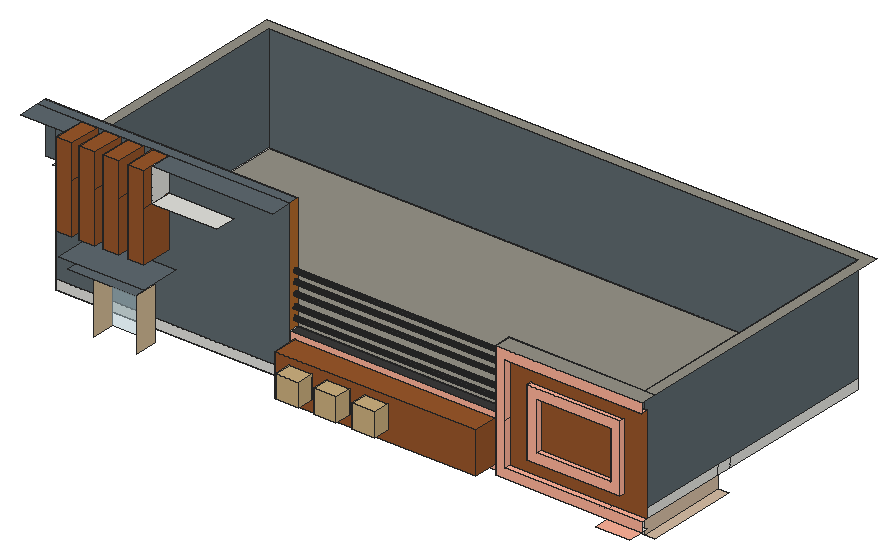
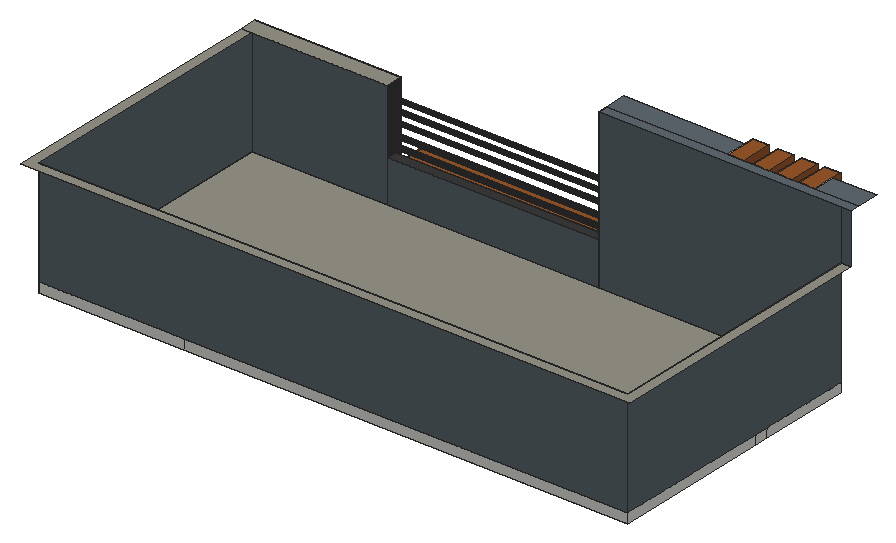
# SketchUp Ruby script. Lengths in inches.
U = 1.inch
M = Sketchup.active_model
def pt(a) = Geom::Point3d.new(a.map { |v| v * U })
def face(e, loops, mat)
  f = e.add_face(loops[0].map { |a| pt(a) })
  loops[1..].each { |l| e.add_face(l.map { |a| pt(a) }).erase! }
  f.material = f.back_material = mat if mat
  f
end
# faces: each face lists its corners as indices into pts; further lists are holes
def faces(e, pts, list, mat = nil) = list.each { |f| face(e, (f[0].is_a?(Array) ? f : [f]).map { |l| l.map { |i| pts[i] } }, mat) }
# xy, xz, yz: faces in a plane at the given z, y or x. An outline is a flat list of corners, or four numbers for a rectangle; further outlines are holes
def ring(l) = l.size == 4 ? [[l[0], l[1]], [l[2], l[1]], [l[2], l[3]], [l[0], l[3]]] : l.each_slice(2).to_a
def flat(e, list, mat, &to3) = list.each { |f| face(e, (f[0].is_a?(Array) ? f : [f]).map { |l| ring(l).map { |u, v| to3.(u, v) } }, mat) }
def xy(e, z, list, mat = nil) = flat(e, list, mat) { |x, y| [x, y, z] }
def xz(e, y, list, mat = nil) = flat(e, list, mat) { |x, z| [x, y, z] }
def yz(e, x, list, mat = nil) = flat(e, list, mat) { |y, z| [x, y, z] }
def lines(e, pts, list) = list.each { |a, b| e.add_line(pt(pts[a]), pt(pts[b])) }
# prism: a flat outline (further loops are holes) pulled along v
def prism(e, loops, v, mat = nil)
  f = face(e, loops, mat); d = Geom::Vector3d.new(v.map { |x| x * U })
  f.pushpull(f.normal.samedirection?(d) ? d.length : -d.length)
end
def box(e, o, s, mat = nil) = prism(e, [[o, [o[0] + s[0], o[1], o[2]], [o[0] + s[0], o[1] + s[1], o[2]], [o[0], o[1] + s[1], o[2]]]], [0, 0, s[2]], mat)
def at(x, y, z, deg = 0) = Geom::Transformation.translation(pt([x, y, z])) * Geom::Transformation.rotation(ORIGIN, Z_AXIS, deg.degrees)
def axes(o, x, y, z) = Geom::Transformation.new([*x, 0, *y, 0, *z, 0, *pt(o).to_a, 1])
def part(name) = M.definitions.add(name)
# library, detail: a bought-in or finely detailed component or shape, given as its bounding box
def library(name, o, s) = part(name).tap { |d| box(d.entities, o, s) }
def detail(e, o, s) = box(e.add_group.entities, o, s)
def put(e, d, t, mat = nil) = e.add_instance(d, t).tap { |i| i.material = mat if mat }
def group(e, t, mat = nil) = e.add_group.tap { |g| g.transformation = t; g.material = mat if mat }.entities
root = M.entities
M.materials.add("[Color B02]").color = [255, 178, 153]
M.materials.add("[Color C02]").color = [255, 204, 153]
M.materials.add("[Color M07]").color = [58, 58, 58]
M.materials.add("[Formica Beige]").color = [211, 187, 149]
M.materials.add("[Formica Graystone]").color = [149, 146, 135]
M.materials.add("[Formica Laminate Light]").color = [213, 189, 164]
M.materials.add("[Formica Speckled Grey]").color = [94, 105, 111]
M.materials.add("[Translucent Glass Safety]").color = [204, 235, 244]
M.materials["[Translucent Glass Safety]"].alpha = 0.5
M.materials.add("[Wood Bamboo]").color = [177, 105, 43]
M.materials.add("[Wood Cherry Original]").color = [152, 86, 42]
M.materials.add("[Wood Floor Light]").color = [204, 176, 127]
xy(root,228.95,[[257.7,166.38,329.95,178.72]])
xy(root,232,[[391.28,166.38,447.72,178.72]])
xy(root,237.86,[[524.83,85.74,533.83,166.38]],"[Formica Laminate Light]")
xy(root,249,[[504.33,70.93,533.83,76.74],[9,166.38,524.83,178.72],[9,178.72,524.83,319.17]])
xy(root,249,[[504.33,57.99,533.83,70.93],[9,85.74,524.83,166.38]],"[Color B02]")
xy(root,249,[[405.9,70.93,405.9,76.74,221.09,76.74,221.09,85.74,504.33,85.74,504.33,70.93]],"[Color C02]")
xy(root,253.72,[[225.3125,54.93,401.17,76.74]],"[Wood Cherry Original]")
xy(root,257.375,[[9,85.74,524.83,319.17]],"[Formica Graystone]")
xy(root,257.39,[[414.29,70.93,504.33,76.74],[504.33,70.93,533.83,76.74]],"[Color B02]")
xy(root,263.47,[[238.12,54.93,258.18,69.68],[271.06,54.93,291.12,69.68],[304.56,54.93,324.62,69.68],[238.12,69.68,258.18,76.74],[271.06,69.68,291.12,76.74],
  [304.56,69.68,324.62,76.74]])
xy(root,263.47,[[238.12,40.06,258.18,54.93],[271.06,40.06,291.12,54.93],[304.56,40.06,324.62,54.93]],"[Wood Floor Light]")
xy(root,269.68,[[432.09,72.56,513.84,76.74]],"[Color B02]")
xy(root,278.24,[[440.64,72.56,505.28,76.74]],"[Color B02]")
xy(root,283.54,[[238.12,54.93,258.18,69.68],[271.06,54.93,291.12,69.68],[304.56,54.93,324.62,69.68],[238.12,69.68,258.18,76.74],[271.06,69.68,291.12,76.74],
  [304.56,69.68,324.62,76.74]])
xy(root,283.54,[[238.12,40.06,258.18,54.93],[271.06,40.06,291.12,54.93],[304.56,40.06,324.62,54.93]],"[Wood Floor Light]")
xy(root,289.38,[[65.18,56.99,102.75,76.74]],"[Formica Beige]")
xy(root,289.78,[[225.3125,54.93,401.17,76.74]],"[Wood Cherry Original]")
xy(root,294.5,[[221.09,76.74,405.9,85.74]],"[Color M07]")
xy(root,300.29,[[54.27,41.68,113.66,56.99]],"[Formica Speckled Grey]")
xy(root,307.5625,[[47,41.68,120.93,76.74]],"[Formica Speckled Grey]")
xy(root,320.12,[[440.64,72.56,505.28,76.74]],"[Color B02]")
xy(root,321.4375,[[38.68,48.99,52.74,76.74],[58.74,48.99,72.8,76.74],[79.11,48.99,93.18,76.74],[100.98,48.99,115.05,76.74]],"[Wood Cherry Original]")
xy(root,328.68,[[432.09,72.56,513.84,76.74]],"[Color B02]")
xy(root,342.48,[[414.29,70.93,533.83,76.74]],"[Color B02]")
xy(root,350.875,[[405.9,70.93,533.83,85.74],[0,85.74,9,85.74,9,319.17,524.83,319.17,524.83,85.74,533.83,85.74,533.83,328.17,0,328.17]],"[Formica Graystone]")
xy(root,365.9375,[[28.26,57.99,38.68,76.74],[115.05,57.99,172.2,76.74]])
xy(root,395.1875,[[0,57.99,38.68,76.74],[115.05,57.99,221.09,76.74],[0,76.74,221.09,85.74]],"[Formica Speckled Grey]")
xy(root,395.1875,[[38.68,48.99,52.74,76.74],[58.74,48.99,72.8,76.74],[79.11,48.99,93.18,76.74],[100.98,48.99,115.05,76.74]],"[Wood Cherry Original]")
xz(root,40.06,[[238.12,263.47,258.18,283.54],[271.06,263.47,291.12,283.54],[304.56,263.47,324.62,283.54]],"[Wood Floor Light]")
xz(root,48.99,[[38.68,321.4375,52.74,395.1875],[58.74,321.4375,72.8,395.1875],[79.11,321.4375,93.18,395.1875],[100.98,321.4375,115.05,395.1875]],"[Wood Cherry Original]")
xz(root,54.93,[[[225.3125,253.72,401.17,289.78],[238.12,263.47,258.18,283.54],[271.06,263.47,291.12,283.54],[304.56,263.47,324.62,283.54]]],"[Wood Cherry Original]")
xz(root,69.68,[[238.12,263.47,258.18,283.54],[271.06,263.47,291.12,283.54],[304.56,263.47,324.62,283.54]])
xz(root,70.93,[[405.9,249,533.83,249,533.83,257.39,414.29,257.39,414.29,342.48,533.83,342.48,533.83,350.875,405.9,350.875]],"[Color B02]")
xz(root,72.56,[[[432.09,269.68,513.84,328.68],[440.64,278.24,505.28,320.12]]],"[Color B02]")
xz(root,76.74,[[238.12,263.47,258.18,283.54],[271.06,263.47,291.12,283.54],[304.56,263.47,324.62,283.54],[38.68,321.4375,52.74,395.1875],[58.74,321.4375,72.8,395.1875],
  [79.11,321.4375,93.18,395.1875],[100.98,321.4375,115.05,395.1875]])
xz(root,76.74,[[[221.09,249,405.9,294.5],[225.3125,253.72,401.17,289.78]]],"[Color B02]")
xz(root,76.74,[[52.74,365.9375,58.74,395.1875],[72.8,365.9375,79.11,395.1875],[93.18,365.9375,100.98,395.1875]],"[Formica Speckled Grey]")
xz(root,76.74,[[65.18,244.12,102.75,289.38]],"[Translucent Glass Safety]")
xz(root,76.74,[[[414.29,257.39,533.83,342.48],[432.09,269.68,513.84,328.68]],[440.64,278.24,505.28,320.12]],"[Wood Cherry Original]")
xz(root,85.74,[[504.33,237.86,524.83,249],[9,249,221.09,257.375],[221.09,249,524.83,257.375]])
xz(root,85.74,[[9,257.375,221.09,395.1875],[221.09,257.375,405.9,294.5],[405.9,257.375,524.83,350.875],[0,350.875,9,395.1875]],"[Formica Speckled Grey]")
xz(root,319.17,[[9,249,398.15,257.375],[398.15,249,524.83,257.375]])
xz(root,319.17,[[9,257.375,524.83,350.875]],"[Formica Speckled Grey]")
yz(root,9,[[85.74,249,166.38,257.375],[166.38,249,178.72,257.375],[178.72,249,319.17,257.375]])
yz(root,9,[[85.74,257.375,319.17,350.875]],"[Formica Speckled Grey]")
yz(root,38.68,[[57.99,365.9375,76.74,395.1875]])
yz(root,38.68,[[48.99,321.4375,76.74,365.9375],[48.99,365.9375,57.99,395.1875]],"[Wood Cherry Original]")
yz(root,52.74,[[48.99,321.4375,76.74,365.9375],[48.99,365.9375,76.74,395.1875]],"[Wood Cherry Original]")
yz(root,58.74,[[48.99,321.4375,76.74,365.9375],[48.99,365.9375,76.74,395.1875]],"[Wood Cherry Original]")
yz(root,65.18,[[56.99,244.12,76.74,289.38]],"[Formica Beige]")
yz(root,72.8,[[48.99,321.4375,76.74,365.9375],[48.99,365.9375,76.74,395.1875]],"[Wood Cherry Original]")
yz(root,79.11,[[48.99,321.4375,76.74,365.9375],[48.99,365.9375,76.74,395.1875]],"[Wood Cherry Original]")
yz(root,93.18,[[48.99,321.4375,76.74,365.9375],[48.99,365.9375,76.74,395.1875]],"[Wood Cherry Original]")
yz(root,100.98,[[48.99,321.4375,76.74,365.9375],[48.99,365.9375,76.74,395.1875]],"[Wood Cherry Original]")
yz(root,102.75,[[56.99,244.12,76.74,289.38]],"[Formica Beige]")
yz(root,115.05,[[57.99,365.9375,76.74,395.1875]])
yz(root,115.05,[[48.99,321.4375,76.74,365.9375],[48.99,365.9375,57.99,395.1875]],"[Wood Cherry Original]")
yz(root,221.09,[[76.74,249,85.74,294.5]])
yz(root,221.09,[[[76.74,294.5,85.74,395.1875],[81.86,301.29,81.42,301.35,81.01,301.52,80.66,301.79,80.39,302.14,80.23,302.54,80.17,302.98,80.23,303.42,80.39,303.82,80.66,304.17,81.01,304.44,81.42,304.61,81.86,304.67,82.29,304.61,82.7,304.44,83.05,304.17,83.32,303.82,83.49,303.42,83.54,302.98,83.49,302.54,83.32,302.14,83.05,301.79,82.7,301.52,82.29,301.35],[81.86,338.61,81.42,338.66,81.01,338.83,80.66,339.1,80.39,339.45,80.23,339.86,80.17,340.29,80.23,340.73,80.39,341.14,80.66,341.49,81.01,341.76,81.42,341.92,81.86,341.98,82.29,341.92,82.7,341.76,83.05,341.49,83.32,341.14,83.49,340.73,83.54,340.29,83.49,339.86,83.32,339.45,83.05,339.1,82.7,338.83,82.29,338.66],[81.86,310.11,81.42,310.16,81.01,310.33,80.66,310.6,80.39,310.95,80.23,311.36,80.17,311.79,80.23,312.23,80.39,312.64,80.66,312.99,81.01,313.26,81.42,313.42,81.86,313.48,82.29,313.42,82.7,313.26,83.05,312.99,83.32,312.64,83.49,312.23,83.54,311.79,83.49,311.36,83.32,310.95,83.05,310.6,82.7,310.33,82.29,310.16],[81.86,329.79,81.42,329.85,81.01,330.02,80.66,330.29,80.39,330.64,80.23,331.04,80.17,331.48,80.23,331.92,80.39,332.32,80.66,332.67,81.01,332.94,81.42,333.11,81.86,333.17,82.29,333.11,82.7,332.94,83.05,332.67,83.32,332.32,83.49,331.92,83.54,331.48,83.49,331.04,83.32,330.64,83.05,330.29,82.7,330.02,82.29,329.85],[81.86,320.61,81.42,320.66,81.01,320.83,80.66,321.1,80.39,321.45,80.23,321.86,80.17,322.29,80.23,322.73,80.39,323.14,80.66,323.49,81.01,323.76,81.42,323.92,81.86,323.98,82.29,323.92,82.7,323.76,83.05,323.49,83.32,323.14,83.49,322.73,83.54,322.29,83.49,321.86,83.32,321.45,83.05,321.1,82.7,320.83,82.29,320.66]]],"[Wood Bamboo]")
yz(root,225.3125,[[54.93,253.72,76.74,289.78]],"[Wood Cherry Original]")
yz(root,238.12,[[54.93,263.47,69.68,283.54],[69.68,263.47,76.74,283.54]])
yz(root,238.12,[[40.06,263.47,54.93,283.54]],"[Wood Floor Light]")
yz(root,258.18,[[54.93,263.47,69.68,283.54],[69.68,263.47,76.74,283.54]])
yz(root,258.18,[[40.06,263.47,54.93,283.54]],"[Wood Floor Light]")
yz(root,271.06,[[54.93,263.47,69.68,283.54],[69.68,263.47,76.74,283.54]])
yz(root,271.06,[[40.06,263.47,54.93,283.54]],"[Wood Floor Light]")
yz(root,291.12,[[54.93,263.47,69.68,283.54],[69.68,263.47,76.74,283.54]])
yz(root,291.12,[[40.06,263.47,54.93,283.54]],"[Wood Floor Light]")
yz(root,304.56,[[54.93,263.47,69.68,283.54],[69.68,263.47,76.74,283.54]])
yz(root,304.56,[[40.06,263.47,54.93,283.54]],"[Wood Floor Light]")
yz(root,324.62,[[54.93,263.47,69.68,283.54],[69.68,263.47,76.74,283.54]])
yz(root,324.62,[[40.06,263.47,54.93,283.54]],"[Wood Floor Light]")
yz(root,401.17,[[54.93,253.72,76.74,289.78]],"[Wood Cherry Original]")
yz(root,405.9,[[81.86,301.29,82.29,301.35,82.7,301.52,83.05,301.79,83.32,302.14,83.49,302.54,83.54,302.98,83.49,303.42,83.32,303.82,83.05,304.17,82.7,304.44,82.29,304.61,81.86,304.67,81.42,304.61,81.01,304.44,80.66,304.17,80.39,303.82,80.23,303.42,80.17,302.98,80.23,302.54,80.39,302.14,80.66,301.79,81.01,301.52,81.42,301.35],[81.86,310.11,82.29,310.16,82.7,310.33,83.05,310.6,83.32,310.95,83.49,311.36,83.54,311.79,83.49,312.23,83.32,312.64,83.05,312.99,82.7,313.26,82.29,313.42,81.86,313.48,81.42,313.42,81.01,313.26,80.66,312.99,80.39,312.64,80.23,312.23,80.17,311.79,80.23,311.36,80.39,310.95,80.66,310.6,81.01,310.33,81.42,310.16],[81.86,320.61,82.29,320.66,82.7,320.83,83.05,321.1,83.32,321.45,83.49,321.86,83.54,322.29,83.49,322.73,83.32,323.14,83.05,323.49,82.7,323.76,82.29,323.92,81.86,323.98,81.42,323.92,81.01,323.76,80.66,323.49,80.39,323.14,80.23,322.73,80.17,322.29,80.23,321.86,80.39,321.45,80.66,321.1,81.01,320.83,81.42,320.66],[81.86,329.79,82.29,329.85,82.7,330.02,83.05,330.29,83.32,330.64,83.49,331.04,83.54,331.48,83.49,331.92,83.32,332.32,83.05,332.67,82.7,332.94,82.29,333.11,81.86,333.17,81.42,333.11,81.01,332.94,80.66,332.67,80.39,332.32,80.23,331.92,80.17,331.48,80.23,331.04,80.39,330.64,80.66,330.29,81.01,330.02,81.42,329.85],[81.86,338.61,82.29,338.66,82.7,338.83,83.05,339.1,83.32,339.45,83.49,339.86,83.54,340.29,83.49,340.73,83.32,341.14,83.05,341.49,82.7,341.76,82.29,341.92,81.86,341.98,81.42,341.92,81.01,341.76,80.66,341.49,80.39,341.14,80.23,340.73,80.17,340.29,80.23,339.86,80.39,339.45,80.66,339.1,81.01,338.83,81.42,338.66]])
yz(root,405.9,[[70.93,249,76.74,294.5],[[70.93,294.5,85.74,350.875],[81.86,338.61,82.29,338.66,82.7,338.83,83.05,339.1,83.32,339.45,83.49,339.86,83.54,340.29,83.49,340.73,83.32,341.14,83.05,341.49,82.7,341.76,82.29,341.92,81.86,341.98,81.42,341.92,81.01,341.76,80.66,341.49,80.39,341.14,80.23,340.73,80.17,340.29,80.23,339.86,80.39,339.45,80.66,339.1,81.01,338.83,81.42,338.66],[81.86,301.29,82.29,301.35,82.7,301.52,83.05,301.79,83.32,302.14,83.49,302.54,83.54,302.98,83.49,303.42,83.32,303.82,83.05,304.17,82.7,304.44,82.29,304.61,81.86,304.67,81.42,304.61,81.01,304.44,80.66,304.17,80.39,303.82,80.23,303.42,80.17,302.98,80.23,302.54,80.39,302.14,80.66,301.79,81.01,301.52,81.42,301.35],[81.86,329.79,82.29,329.85,82.7,330.02,83.05,330.29,83.32,330.64,83.49,331.04,83.54,331.48,83.49,331.92,83.32,332.32,83.05,332.67,82.7,332.94,82.29,333.11,81.86,333.17,81.42,333.11,81.01,332.94,80.66,332.67,80.39,332.32,80.23,331.92,80.17,331.48,80.23,331.04,80.39,330.64,80.66,330.29,81.01,330.02,81.42,329.85],[81.86,310.11,82.29,310.16,82.7,310.33,83.05,310.6,83.32,310.95,83.49,311.36,83.54,311.79,83.49,312.23,83.32,312.64,83.05,312.99,82.7,313.26,82.29,313.42,81.86,313.48,81.42,313.42,81.01,313.26,80.66,312.99,80.39,312.64,80.23,312.23,80.17,311.79,80.23,311.36,80.39,310.95,80.66,310.6,81.01,310.33,81.42,310.16],[81.86,320.61,82.29,320.66,82.7,320.83,83.05,321.1,83.32,321.45,83.49,321.86,83.54,322.29,83.49,322.73,83.32,323.14,83.05,323.49,82.7,323.76,82.29,323.92,81.86,323.98,81.42,323.92,81.01,323.76,80.66,323.49,80.39,323.14,80.23,322.73,80.17,322.29,80.23,321.86,80.39,321.45,80.66,321.1,81.01,320.83,81.42,320.66]]],"[Color M07]")
yz(root,414.29,[[70.93,257.39,76.74,294.5],[70.93,294.5,76.74,342.48]],"[Color B02]")
yz(root,432.09,[[72.56,269.68,76.74,328.68]],"[Color B02]")
yz(root,440.64,[[72.56,278.24,76.74,320.12]],"[Color B02]")
yz(root,505.28,[[72.56,278.24,76.74,320.12]],"[Color B02]")
yz(root,513.84,[[72.56,269.68,76.74,328.68]],"[Color B02]")
yz(root,524.83,[[85.74,249,166.38,257.375],[166.38,249,178.72,257.375],[178.72,249,319.17,257.375]])
yz(root,524.83,[[85.74,237.86,166.38,249]],"[Formica Laminate Light]")
yz(root,524.83,[[85.74,257.375,319.17,350.875]],"[Formica Speckled Grey]")
p = [[405.9,81.86,301.29],[405.9,81.42,301.35],[221.09,81.42,301.35],[221.09,81.86,301.29],[405.9,82.29,301.35],[221.09,82.29,301.35],
  [405.9,81.01,301.52],[221.09,81.01,301.52],[405.9,82.7,301.52],[221.09,82.7,301.52],[405.9,80.66,301.79],[221.09,80.66,301.79],
  [405.9,83.05,301.79],[221.09,83.05,301.79],[405.9,80.39,302.14],[221.09,80.39,302.14],[405.9,83.32,302.14],[221.09,83.32,302.14],
  [405.9,80.23,302.54],[221.09,80.23,302.54],[405.9,83.49,302.54],[221.09,83.49,302.54],[405.9,80.17,302.98],[221.09,80.17,302.98],
  [405.9,83.54,302.98],[221.09,83.54,302.98],[405.9,80.23,303.42],[221.09,80.23,303.42],[405.9,83.49,303.42],[221.09,83.49,303.42],
  [405.9,80.39,303.82],[221.09,80.39,303.82],[405.9,83.32,303.82],[221.09,83.32,303.82],[405.9,80.66,304.17],[221.09,80.66,304.17],
  [405.9,83.05,304.17],[221.09,83.05,304.17],[405.9,81.01,304.44],[221.09,81.01,304.44],[405.9,82.7,304.44],[221.09,82.7,304.44],
  [405.9,81.42,304.61],[221.09,81.42,304.61],[405.9,82.29,304.61],[221.09,82.29,304.61],[405.9,81.86,304.67],[221.09,81.86,304.67],
  [405.9,81.86,310.11],[405.9,81.42,310.16],[221.09,81.42,310.16],[221.09,81.86,310.11],[405.9,82.29,310.16],[221.09,82.29,310.16],
  [405.9,81.01,310.33],[221.09,81.01,310.33],[405.9,82.7,310.33],[221.09,82.7,310.33],[405.9,80.66,310.6],[221.09,80.66,310.6],
  [405.9,83.05,310.6],[221.09,83.05,310.6],[405.9,80.39,310.95],[221.09,80.39,310.95],[405.9,83.32,310.95],[221.09,83.32,310.95],
  [405.9,80.23,311.36],[221.09,80.23,311.36],[405.9,83.49,311.36],[221.09,83.49,311.36],[405.9,80.17,311.79],[221.09,80.17,311.79],
  [405.9,83.54,311.79],[221.09,83.54,311.79],[405.9,80.23,312.23],[221.09,80.23,312.23],[405.9,83.49,312.23],[221.09,83.49,312.23],
  [405.9,80.39,312.64],[221.09,80.39,312.64],[405.9,83.32,312.64],[221.09,83.32,312.64],[405.9,80.66,312.99],[221.09,80.66,312.99],
  [405.9,83.05,312.99],[221.09,83.05,312.99],[405.9,81.01,313.26],[221.09,81.01,313.26],[405.9,82.7,313.26],[221.09,82.7,313.26],
  [405.9,81.42,313.42],[221.09,81.42,313.42],[405.9,82.29,313.42],[221.09,82.29,313.42],[405.9,81.86,313.48],[221.09,81.86,313.48],
  [405.9,81.86,320.61],[405.9,81.42,320.66],[221.09,81.42,320.66],[221.09,81.86,320.61],[405.9,82.29,320.66],[221.09,82.29,320.66],
  [405.9,81.01,320.83],[221.09,81.01,320.83],[405.9,82.7,320.83],[221.09,82.7,320.83],[405.9,80.66,321.1],[221.09,80.66,321.1],
  [405.9,83.05,321.1],[221.09,83.05,321.1],[405.9,80.39,321.45],[221.09,80.39,321.45],[405.9,83.32,321.45],[221.09,83.32,321.45],
  [405.9,80.23,321.86],[221.09,80.23,321.86],[405.9,83.49,321.86],[221.09,83.49,321.86],[405.9,80.17,322.29],[221.09,80.17,322.29],
  [405.9,83.54,322.29],[221.09,83.54,322.29],[405.9,80.23,322.73],[221.09,80.23,322.73],[405.9,83.49,322.73],[221.09,83.49,322.73],
  [405.9,80.39,323.14],[221.09,80.39,323.14],[405.9,83.32,323.14],[221.09,83.32,323.14],[405.9,80.66,323.49],[221.09,80.66,323.49],
  [405.9,83.05,323.49],[221.09,83.05,323.49],[405.9,81.01,323.76],[221.09,81.01,323.76],[405.9,82.7,323.76],[221.09,82.7,323.76],
  [405.9,81.42,323.92],[221.09,81.42,323.92],[405.9,82.29,323.92],[221.09,82.29,323.92],[405.9,81.86,323.98],[221.09,81.86,323.98],
  [405.9,81.86,329.79],[405.9,81.42,329.85],[221.09,81.42,329.85],[221.09,81.86,329.79],[405.9,82.29,329.85],[221.09,82.29,329.85],
  [405.9,81.01,330.02],[221.09,81.01,330.02],[405.9,82.7,330.02],[221.09,82.7,330.02],[405.9,80.66,330.29],[221.09,80.66,330.29],
  [405.9,83.05,330.29],[221.09,83.05,330.29],[405.9,80.39,330.64],[221.09,80.39,330.64],[405.9,83.32,330.64],[221.09,83.32,330.64],
  [405.9,80.23,331.04],[221.09,80.23,331.04],[405.9,83.49,331.04],[221.09,83.49,331.04],[405.9,80.17,331.48],[221.09,80.17,331.48],
  [405.9,83.54,331.48],[221.09,83.54,331.48],[405.9,80.23,331.92],[221.09,80.23,331.92],[405.9,83.49,331.92],[221.09,83.49,331.92],
  [405.9,80.39,332.32],[221.09,80.39,332.32],[405.9,83.32,332.32],[221.09,83.32,332.32],[405.9,80.66,332.67],[221.09,80.66,332.67],
  [405.9,83.05,332.67],[221.09,83.05,332.67],[405.9,81.01,332.94],[221.09,81.01,332.94],[405.9,82.7,332.94],[221.09,82.7,332.94],
  [405.9,81.42,333.11],[221.09,81.42,333.11],[405.9,82.29,333.11],[221.09,82.29,333.11],[405.9,81.86,333.17],[221.09,81.86,333.17],
  [405.9,81.86,338.61],[405.9,81.42,338.66],[221.09,81.42,338.66],[221.09,81.86,338.61],[405.9,82.29,338.66],[221.09,82.29,338.66],
  [405.9,81.01,338.83],[221.09,81.01,338.83],[405.9,82.7,338.83],[221.09,82.7,338.83],[405.9,80.66,339.1],[221.09,80.66,339.1],
  [405.9,83.05,339.1],[221.09,83.05,339.1],[405.9,80.39,339.45],[221.09,80.39,339.45],[405.9,83.32,339.45],[221.09,83.32,339.45],
  [405.9,80.23,339.86],[221.09,80.23,339.86],[405.9,83.49,339.86],[221.09,83.49,339.86],[405.9,80.17,340.29],[221.09,80.17,340.29],
  [405.9,83.54,340.29],[221.09,83.54,340.29],[405.9,80.23,340.73],[221.09,80.23,340.73],[405.9,83.49,340.73],[221.09,83.49,340.73],
  [405.9,80.39,341.14],[221.09,80.39,341.14],[405.9,83.32,341.14],[221.09,83.32,341.14],[405.9,80.66,341.49],[221.09,80.66,341.49],
  [405.9,83.05,341.49],[221.09,83.05,341.49],[405.9,81.01,341.76],[221.09,81.01,341.76],[405.9,82.7,341.76],[221.09,82.7,341.76],
  [405.9,81.42,341.92],[221.09,81.42,341.92],[405.9,82.29,341.92],[221.09,82.29,341.92],[405.9,81.86,341.98],[221.09,81.86,341.98]]
faces(root,p,[[0,1,2,3],[4,0,3,5],[1,6,7,2],[8,4,5,9],[6,10,11,7],[12,8,9,13],[10,14,15,11],[16,12,13,17],
  [14,18,19,15],[20,16,17,21],[18,22,23,19],[24,20,21,25],[22,26,27,23],[28,24,25,29],[26,30,31,27],[32,28,29,33],
  [30,34,35,31],[36,32,33,37],[34,38,39,35],[40,36,37,41],[38,42,43,39],[44,40,41,45],[42,46,47,43],[46,44,45,47],
  [48,49,50,51],[52,48,51,53],[49,54,55,50],[56,52,53,57],[54,58,59,55],[60,56,57,61],[58,62,63,59],[64,60,61,65],
  [62,66,67,63],[68,64,65,69],[66,70,71,67],[72,68,69,73],[70,74,75,71],[76,72,73,77],[74,78,79,75],[80,76,77,81],
  [78,82,83,79],[84,80,81,85],[82,86,87,83],[88,84,85,89],[86,90,91,87],[92,88,89,93],[90,94,95,91],[94,92,93,95],
  [96,97,98,99],[100,96,99,101],[97,102,103,98],[104,100,101,105],[102,106,107,103],[108,104,105,109],[106,110,111,107],[112,108,109,113],
  [110,114,115,111],[116,112,113,117],[114,118,119,115],[120,116,117,121],[118,122,123,119],[124,120,121,125],[122,126,127,123],[128,124,125,129],
  [126,130,131,127],[132,128,129,133],[130,134,135,131],[136,132,133,137],[134,138,139,135],[140,136,137,141],[138,142,143,139],[142,140,141,143],
  [144,145,146,147],[148,144,147,149],[145,150,151,146],[152,148,149,153],[150,154,155,151],[156,152,153,157],[154,158,159,155],[160,156,157,161],
  [158,162,163,159],[164,160,161,165],[162,166,167,163],[168,164,165,169],[166,170,171,167],[172,168,169,173],[170,174,175,171],[176,172,173,177],
  [174,178,179,175],[180,176,177,181],[178,182,183,179],[184,180,181,185],[182,186,187,183],[188,184,185,189],[186,190,191,187],[190,188,189,191],
  [192,193,194,195],[196,192,195,197],[193,198,199,194],[200,196,197,201],[198,202,203,199],[204,200,201,205],[202,206,207,203],[208,204,205,209],
  [206,210,211,207],[212,208,209,213],[210,214,215,211],[216,212,213,217],[214,218,219,215],[220,216,217,221],[218,222,223,219],[224,220,221,225],
  [222,226,227,223],[228,224,225,229],[226,230,231,227],[232,228,229,233],[230,234,235,231],[236,232,233,237],[234,238,239,235],[238,236,237,239]],"[Color M07]")
